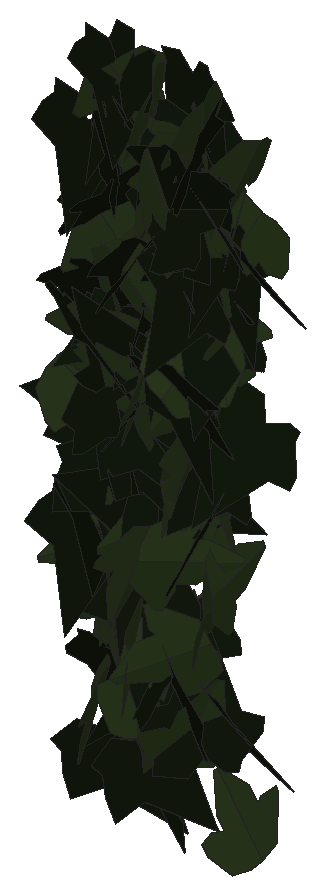
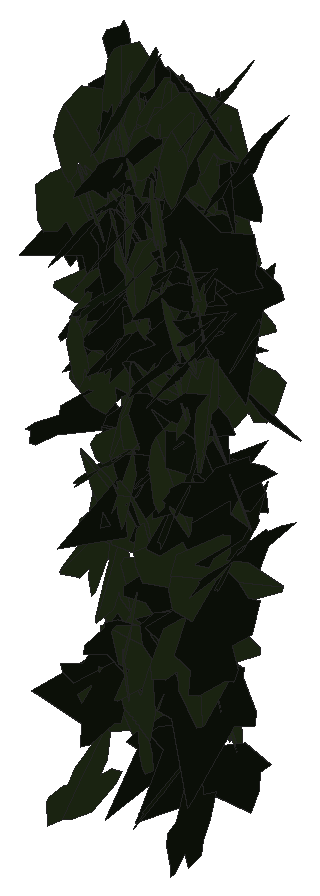
# SketchUp Ruby script. Lengths in inches.
U = 1.inch
M = Sketchup.active_model
def pt(a) = Geom::Point3d.new(a.map { |v| v * U })
def face(e, loops, mat)
  f = e.add_face(loops[0].map { |a| pt(a) })
  loops[1..].each { |l| e.add_face(l.map { |a| pt(a) }).erase! }
  f.material = f.back_material = mat if mat
  f
end
# faces: each face lists its corners as indices into pts; further lists are holes
def faces(e, pts, list, mat = nil) = list.each { |f| face(e, (f[0].is_a?(Array) ? f : [f]).map { |l| l.map { |i| pts[i] } }, mat) }
# xy, xz, yz: faces in a plane at the given z, y or x. An outline is a flat list of corners, or four numbers for a rectangle; further outlines are holes
def ring(l) = l.size == 4 ? [[l[0], l[1]], [l[2], l[1]], [l[2], l[3]], [l[0], l[3]]] : l.each_slice(2).to_a
def flat(e, list, mat, &to3) = list.each { |f| face(e, (f[0].is_a?(Array) ? f : [f]).map { |l| ring(l).map { |u, v| to3.(u, v) } }, mat) }
def xy(e, z, list, mat = nil) = flat(e, list, mat) { |x, y| [x, y, z] }
def xz(e, y, list, mat = nil) = flat(e, list, mat) { |x, z| [x, y, z] }
def yz(e, x, list, mat = nil) = flat(e, list, mat) { |y, z| [x, y, z] }
def lines(e, pts, list) = list.each { |a, b| e.add_line(pt(pts[a]), pt(pts[b])) }
# prism: a flat outline (further loops are holes) pulled along v
def prism(e, loops, v, mat = nil)
  f = face(e, loops, mat); d = Geom::Vector3d.new(v.map { |x| x * U })
  f.pushpull(f.normal.samedirection?(d) ? d.length : -d.length)
end
def box(e, o, s, mat = nil) = prism(e, [[o, [o[0] + s[0], o[1], o[2]], [o[0] + s[0], o[1] + s[1], o[2]], [o[0], o[1] + s[1], o[2]]]], [0, 0, s[2]], mat)
def at(x, y, z, deg = 0) = Geom::Transformation.translation(pt([x, y, z])) * Geom::Transformation.rotation(ORIGIN, Z_AXIS, deg.degrees)
def axes(o, x, y, z) = Geom::Transformation.new([*x, 0, *y, 0, *z, 0, *pt(o).to_a, 1])
def part(name) = M.definitions.add(name)
# library, detail: a bought-in or finely detailed component or shape, given as its bounding box
def library(name, o, s) = part(name).tap { |d| box(d.entities, o, s) }
def detail(e, o, s) = box(e.add_group.entities, o, s)
def put(e, d, t, mat = nil) = e.add_instance(d, t).tap { |i| i.material = mat if mat }
def group(e, t, mat = nil) = e.add_group.tap { |g| g.transformation = t; g.material = mat if mat }.entities
root = M.entities
M.materials.add("efeu1").color = [18, 25, 13]
M.materials.add("efeu2").color = [43, 57, 29]
c1 = part("ivyleaf_10")
p = [[0,0.5,-0.03],[-0.0625,2.02,-0.43],[-0.19,2.01,-0.46],[-0.54,1.05,-0.29],[-0.52,0.625,-0.18],[-0.83,0.76,-0.28],
  [-1.16,0.64,-0.33],[-1.15,0.33,-0.24],[-0.77,-0.39,0.02],[-0.3,-0.51,0.16],[0.04,-0.48,0.23],[-0.02,2.01,-0.4375],
  [-0.06,2.01,-0.43],[0.04,-0.49,0.23],[0.67,-0.49,0.14],[1.38,0.36,-0.2],[1.375,0.51,-0.24],[0.81,0.65,-0.19],
  [0.62,0.59,-0.15],[0.6,1.09,-0.28],[0.5,1.23,-0.31]]
faces(c1.entities,p,[[0,1,2,3,4,5,6,7,8,9,10],[11,12,0,13,14,15,16,17,18,19,20]],"efeu2")
c2 = part("ivyleaf_9")
p = [[1.54,2.16,1.25],[1.36,2.04,1.19],[-0.21,0.99,0.68],[-0.71,1.11,0.82],[-0.85,0.86,0.67],[-0.8,0.17,0.21],
  [-0.9,-0.01,0.1],[-0.67,-0.16,-0.02],[-0.08,-0.08,-0.05],[-0.03,-0.6,-0.4],[0.65,-0.88,-0.66],[0.83,-0.6,-0.49],
  [1.29,-0.42,-0.43],[1.8125,-0.07,-0.26],[1.21,0.44,0.15]]
faces(c2.entities,p,[[0,1,2,3,4,5,6,7,8,9,10,11,12,13,14]],"efeu1")
put(root,c1,axes([25.92,223.86,216.84],[-0.09264,-0.02224,0.49084],[-0.23134,-0.43869,-0.06354],[0.43347,-0.23887,0.07099]))
put(root,c2,axes([25.3,224.02,216.3125],[0.30495,-0.20069,0.34166],[0.2981,-0.16782,-0.36465],[0.26104,0.4261,0.01729]))
put(root,c1,axes([25.88,223.6875,219.36],[-0.37666,0.25048,0.21305],[-0.18134,0.11202,-0.45229],[-0.27431,-0.41799,0.00646]))
put(root,c2,axes([25.625,223.57,217.05],[-0.07559,-0.47947,0.11996],[0.00181,-0.12162,-0.48498],[0.49425,-0.07289,0.02013]))
put(root,c2,axes([25.65,224.01,218.25],[-0.14085,-0.47505,-0.06702],[0.02033,0.06387,-0.49549],[0.47932,-0.1423,0.00132]))
put(root,c2,axes([25.6,223.5,222.08],[0.01946,-0.45872,0.19799],[-0.01144,-0.1985,-0.45877],[0.49949,0.01332,-0.01821]))
put(root,c1,axes([25.62,223.44,217.71],[0.39091,-0.27001,-0.15584],[0.13229,-0.08265,0.47504],[-0.28229,-0.41263,0.00682]))
put(root,c1,axes([25.9,223.83,216.08],[-0.29931,-0.40022,0.01555],[-0.00929,-0.01247,-0.49976],[0.40041,-0.29945,0.00003]))
put(root,c2,axes([25.69,223.82,220.875],[-0.28485,0.05445,0.4073],[0.37648,-0.16405,0.28523],[0.16469,0.46917,0.05246]))
put(root,c2,axes([25.61,223.53,217.14],[0.09476,-0.35196,0.34226],[0.0888,-0.33054,-0.3645],[0.48284,0.12987,-0.00014]))
put(root,c2,axes([25.72,224.27,213.65],[-0.14512,-0.03935,0.47685],[0.10819,-0.4881,-0.00735],[0.46608,0.10104,0.15019]))
put(root,c2,axes([25.9,223.6,215.45],[0.37979,0.21595,-0.24315],[-0.21529,-0.11324,-0.43684],[-0.24374,0.43651,0.00697]))
put(root,c2,axes([26.05,223.25,220.45],[0.16703,0.37187,-0.28951],[-0.19296,-0.22627,-0.40196],[-0.42996,0.24601,0.06793]))
put(root,c1,axes([25.74,223.08,219.14],[0.21945,0.31613,0.31922],[0.11666,0.30299,-0.38025],[-0.43386,0.24137,0.05923]))
put(root,c1,axes([25.95,223.31,215.2],[0.24757,-0.43141,0.05097],[0.02373,-0.04514,-0.49739],[0.43376,0.2487,-0.00187]))
put(root,c2,axes([26.36,223.02,219.06],[-0.32886,0.23102,0.29746],[-0.26211,0.14319,-0.40099],[-0.27046,-0.41967,0.02693]))
put(root,c1,axes([25.99,223.97,222.44],[-0.01091,-0.44648,0.2248],[0.04308,-0.22486,-0.4445],[0.49802,0.00967,0.04338]))
put(root,c2,axes([25.69,223.09,220.02],[0.39503,-0.30608,0.01632],[0.01447,-0.00797,-0.49973],[0.30617,0.39529,0.00256]))
put(root,c2,axes([26.26,223.05,222.3125],[0.07939,0.0261,-0.49297],[-0.49223,0.04213,-0.07704],[0.03752,0.49754,0.03239]))
put(root,c1,axes([25.94,223.7,222.73],[-0.29531,-0.32227,-0.24277],[0.16607,0.1771,-0.4371],[0.36771,-0.3388,0.00244]))
put(root,c1,axes([26.03,223.42,220.59],[-0.25135,0.42248,0.09129],[-0.05371,0.07425,-0.49153],[-0.42888,-0.2569,0.00806]))
put(root,c1,axes([26.05,223.84,220.99],[0.3085,-0.38628,-0.07493],[-0.03814,0.06541,-0.49423],[0.39163,0.31066,0.0109]))
put(root,c2,axes([25.83,224.07,219.8125],[0.07503,-0.48177,0.11074],[0.01907,-0.1091,-0.48758],[0.49397,0.07739,0.002]))
put(root,c2,axes([25.86,223.98,220.7],[0.02957,-0.45823,-0.19786],[0.0326,0.19956,-0.45729],[0.49806,0.01414,0.04168]))
put(root,c1,axes([26.02,224.14,220.49],[0.23063,-0.41696,0.15151],[0.07045,-0.13417,-0.47648],[0.43801,0.24113,-0.00314]))
put(root,c2,axes([26.1,223.83,217.34],[0.37924,-0.03383,0.32409],[-0.32081,0.04835,0.38045],[-0.05708,-0.49651,0.01496]))
put(root,c2,axes([26.09,223.71,222.96],[-0.4266,0.00649,-0.26071],[0.26023,-0.02229,-0.42636],[-0.01716,-0.49946,0.01564]))
put(root,c2,axes([25.86,223.76,222.76],[0.02824,-0.4353,0.24438],[0.07206,-0.23865,-0.43342],[0.49397,0.0597,0.04926]))
put(root,c1,axes([26.2,223.11,219.92],[-0.45447,-0.18164,0.10227],[-0.08785,-0.05557,-0.48908],[0.18904,-0.46251,0.0186]))
put(root,c2,axes([26.26,224.04,219.85],[-0.33124,-0.26273,0.26693],[-0.18906,-0.19032,-0.42194],[0.32332,-0.38046,0.02674]))
put(root,c1,axes([26.15,224.08,218.45],[0.0985,-0.48186,0.09004],[0.01335,-0.08917,-0.4918],[0.49002,0.09929,-0.0047]))
put(root,c2,axes([25.96,224.16,217.85],[0.02168,-0.23686,0.4398],[0.05246,-0.4367,-0.23778],[0.49677,0.05645,0.00592]))
put(root,c1,axes([26.07,223.32,221.05],[-0.23934,-0.38368,-0.21332],[0.20248,0.11909,-0.44138],[0.38951,-0.29766,0.09837]))
put(root,c2,axes([25.93,223.46,214.49],[-0.09453,-0.15668,-0.46531],[0.22631,0.40661,-0.1829],[0.43572,-0.24518,-0.00596]))
put(root,c1,axes([25.88,223.52,216.28],[0.1338,-0.13367,0.46285],[0.40176,-0.23413,-0.18376],[0.26586,0.42109,0.04475]))
put(root,c2,axes([26.1,224.24,219.74],[-0.12442,-0.41104,0.25605],[-0.01447,-0.2611,-0.42617],[0.48405,-0.11346,0.05308]))
put(root,c2,axes([26.33,223.99,220.51],[-0.38732,-0.29247,0.12021],[-0.08899,-0.08158,-0.48521],[0.30343,-0.39725,0.01114]))
put(root,c2,axes([26.28,222.98,221.65],[0.11209,0.48323,0.06269],[0.01307,0.06132,-0.49605],[-0.4871,0.11284,0.00112]))
put(root,c2,axes([26.04,223.44,218.04],[-0.17073,-0.30697,-0.35584],[0.1756,0.3095,-0.35125],[0.43591,-0.24491,0.00213]))
put(root,c2,axes([25.92,223.86,222.29],[0.36282,-0.33171,0.09129],[0.06779,-0.06114,-0.4916],[0.3373,0.36909,0.00061]))
put(root,c1,axes([26.4,223.13,219.41],[-0.46056,-0.14243,0.13267],[-0.12576,-0.04237,-0.48207],[0.14857,-0.47741,0.0032]))
put(root,c2,axes([26.43,223.75,217.41],[-0.01959,-0.017,0.49933],[-0.41095,-0.28365,-0.02578],[0.28415,-0.4114,-0.00286]))
put(root,c1,axes([26.46,223.62,222.21],[-0.44911,-0.17426,0.13391],[-0.1138,-0.07624,-0.48087],[0.18801,-0.46241,0.02882]))
put(root,c2,axes([26.07,224,214.35],[0.21511,-0.45076,0.02334],[0.01062,-0.0208,-0.49945],[0.45124,0.21537,0.00062]))
put(root,c1,axes([26.39,223.86,220.82],[-0.07417,-0.47008,0.15338],[0.01785,-0.15754,-0.4742],[0.49415,-0.06487,0.04015]))
put(root,c1,axes([26.05,223.64,214.33],[-0.18337,0.00872,0.46508],[0.43547,-0.17253,0.17493],[0.16353,0.46921,0.05568]))
put(root,c2,axes([26.23,223.35,218.46],[-0.04078,0.49826,0.00887],[-0.00261,-0.00912,0.49991],[0.49833,0.04072,0.00335]))
put(root,c1,axes([26.41,223.96,217.15],[-0.02506,0.01961,0.49899],[0.01468,-0.49937,0.02036],[0.49916,0.01567,0.02446]))
put(root,c1,axes([26.46,223.56,222.65],[0.09237,-0.40977,-0.27122],[-0.02638,0.27144,-0.41908],[0.49068,0.09173,0.02852]))
put(root,c2,axes([26.28,223.91,218.97],[-0.19526,-0.37314,-0.26952],[0.11483,0.24402,-0.42103],[0.44574,-0.22632,-0.0096]))
put(root,c1,axes([26.46,223.52,218.66],[-0.33117,0.37288,0.03585],[0.02405,-0.02659,0.49871],[0.37383,0.33204,-0.00032]))
put(root,c2,axes([26.57,223.3,219.23],[0.25555,0.00267,0.42975],[-0.42824,0.04361,0.25438],[-0.03612,-0.49809,0.02457]))
put(root,c2,axes([26.34,223.63,216.52],[-0.32198,-0.29113,-0.24814],[0.17468,0.17665,-0.43391],[0.34032,-0.36611,-0.01205]))
put(root,c1,axes([26.47,223.8,221.51],[0.16813,-0.45372,-0.12599],[-0.04098,0.11917,-0.48386],[0.4691,0.17303,0.00289]))
put(root,c2,axes([26.68,223.45,215.59],[-0.43694,0.2318,-0.07316],[0.06226,-0.03874,-0.49459],[-0.23496,-0.44132,0.00498]))
put(root,c1,axes([26.31,223.52,215.95],[0.23028,-0.31621,0.31142],[0.21559,-0.22696,-0.38988],[0.38793,0.31385,0.03181]))
put(root,c1,axes([26.47,223.41,219.17],[0.23988,-0.43815,0.02189],[0.00612,-0.0216,-0.4995],[0.43866,0.2399,-0.005]))
put(root,c2,axes([26.625,223.01,220.82],[-0.0202,0.45126,0.21438],[0.00085,0.21459,-0.45161],[-0.49959,-0.01788,-0.00944]))
put(root,c1,axes([26.53,223.33,217.15],[0.01692,-0.46884,0.17292],[0.01414,-0.1725,-0.46909],[0.49951,0.02076,0.00743]))
put(root,c1,axes([26.55,223.16,215.08],[-0.01082,0.46922,-0.17239],[-0.00378,0.17235,0.46934],[0.49987,0.01146,-0.00019]))
put(root,c2,axes([26.29,223.58,218.33],[0.2317,-0.39063,-0.20909],[-0.0385,0.21731,-0.44866],[0.4414,0.22401,0.07062]))
put(root,c1,axes([26.54,224.07,220.61],[0.15258,-0.38364,0.28203],[0.10313,-0.2625,-0.41287],[0.46485,0.18416,-0.00098]))
put(root,c1,axes([26.625,223.44,221.58],[-0.47344,0.15701,-0.03462],[0.03459,-0.00567,-0.49877],[-0.15702,-0.47467,-0.00549]))
put(root,c2,axes([26.47,223.36,214.57],[0.12144,-0.26162,-0.40842],[-0.07568,0.40565,-0.28235],[0.47909,0.13039,0.05893]))
put(root,c2,axes([26.79,223.17,221.09],[0.04507,0.44037,-0.23248],[-0.03539,-0.23001,-0.44254],[-0.49671,0.05635,0.01043]))
put(root,c2,axes([26.36,224.09,220.58],[0.10427,-0.31253,0.3761],[0.16457,-0.3397,-0.3279],[0.46049,0.19217,0.03202]))
put(root,c1,axes([26.48,223.04,220.85],[-0.40393,0.0784,-0.28407],[0.27901,-0.0534,-0.41147],[-0.09486,-0.49092,-0.00061]))
put(root,c2,axes([26.5,223.45,218.78],[0.00831,-0.34951,-0.35746],[0.05502,0.35597,-0.34678],[0.49689,-0.03357,0.04437]))
put(root,c2,axes([26.51,223.9,219.87],[0.13072,-0.44339,-0.19057],[-0.02937,0.18976,-0.46166],[0.48172,0.13189,0.02357]))
put(root,c2,axes([26.46,223.61,217.76],[0.04818,-0.01555,-0.49743],[0.1009,0.48968,-0.00554],[0.48734,-0.09985,0.05032]))
put(root,c1,axes([26.37,224.14,214.84],[0.01469,-0.07094,0.49472],[0.46274,-0.18507,-0.04027],[0.18883,0.45904,0.06022]))
put(root,c2,axes([26.625,223.94,216.01],[-0.21428,-0.41987,-0.16672],[0.0709,0.15098,-0.47136],[0.44616,-0.22564,-0.00517]))
put(root,c1,axes([26.67,223.54,215.5],[0.14754,0.28275,-0.38508],[0.12259,0.36712,0.31653],[0.46174,-0.18781,0.039]))
put(root,c1,axes([26.62,224.05,218.85],[-0.10077,-0.03125,0.48874],[0.2207,-0.44834,0.01684],[0.43719,0.21913,0.10415]))
put(root,c1,axes([27.11,224.12,219.45],[-0.13771,-0.10106,0.46992],[-0.37913,-0.27764,-0.17081],[0.29546,-0.40337,-0.00016]))
put(root,c2,axes([26.6,223.5,220.09],[-0.01149,-0.04789,-0.49757],[0.1108,0.48508,-0.04924],[0.48743,-0.11139,-0.00054]))
put(root,c1,axes([26.87,223.49,221.99],[0.03217,-0.44888,0.21788],[-0.00197,-0.21844,-0.44975],[0.49896,0.02808,-0.01582]))
put(root,c2,axes([26.64,223.91,219.78],[0.05427,-0.47739,-0.13839],[0.00108,0.13932,-0.4802],[0.49705,0.05182,0.01615]))
put(root,c1,axes([26.72,224.07,219.0625],[-0.125,0.33887,-0.34574],[0.07489,-0.33925,-0.35958],[-0.4783,-0.14168,0.03406]))
put(root,c2,axes([26.79,224.35,220.42],[-0.21873,-0.28318,0.34923],[0.02701,-0.39594,-0.30414],[0.44881,-0.11419,0.1885]))
put(root,c2,axes([26.7,224.11,222.15],[-0.02224,-0.49506,-0.06647],[0.01144,0.06602,-0.49549],[0.49937,-0.02356,0.00839]))
put(root,c2,axes([26.7,223.93,220.4],[0.1171,-0.4854,-0.02586],[-0.00057,0.02647,-0.4993],[0.48609,0.11697,0.00565]))
put(root,c1,axes([26.63,224.18,215.75],[0.02832,-0.10785,0.48741],[0.39932,-0.28807,-0.08694],[0.29957,0.39419,0.06982]))
put(root,c1,axes([27.21,223.375,216.03],[-0.1742,-0.13423,0.44904],[-0.3376,-0.29636,-0.21955],[0.32509,-0.37968,0.01262]))
put(root,c2,axes([27.03,223.6,220.99],[-0.14488,0.33229,-0.34438],[0.13202,-0.3181,-0.36247],[-0.45998,-0.19596,0.00443]))
put(root,c1,axes([27.04,222.9,222.27],[-0.11141,0.44621,0.19617],[-0.12853,0.16721,-0.45334],[-0.47018,-0.15144,0.07745]))
put(root,c2,axes([26.73,224.02,222.83],[0.22354,-0.43653,0.09733],[0.03063,-0.09361,-0.4902],[0.4462,0.22512,-0.01511]))
put(root,c1,axes([26.67,224.05,217.39],[0.25981,-0.13375,-0.40572],[0.37364,-0.15906,0.2917],[-0.2071,-0.45477,0.0173]))
put(root,c2,axes([26.79,223.85,221.19],[0.27173,-0.39147,-0.15138],[-0.04405,0.15274,-0.47406],[0.4174,0.27097,0.04852]))
put(root,c1,axes([27,223.7,222.23],[0.23688,-0.42763,0.10497],[0.05135,-0.09155,-0.48886],[0.43732,0.24238,0.00055]))
put(root,c1,axes([26.91,223.96,218.03],[-0.36664,0.27092,-0.20537],[0.16535,-0.12181,-0.45588],[-0.29705,-0.4022,-0.00027]))
put(root,c1,axes([27.19,223.08,218.3],[-0.07843,0.1704,0.46348],[-0.24243,0.39556,-0.18645],[-0.43021,-0.25396,0.02058]))
put(root,c2,axes([27.51,223.08,221.58],[-0.2086,0.23029,0.39173],[-0.32546,0.22509,-0.30564],[-0.31712,-0.38249,0.05599]))
put(root,c1,axes([27.45,223.69,221.12],[-0.14269,0.09933,0.4688],[-0.44746,0.14745,-0.16744],[-0.17151,-0.46732,0.04681]))
put(root,c2,axes([27.04,224.03,218.04],[-0.18763,-0.36123,0.29036],[0.05837,-0.32917,-0.3718],[0.45977,-0.10562,0.16569]))
put(root,c2,axes([27.41,223.01,222.31],[0.14569,0.22809,-0.42042],[-0.35729,-0.24029,-0.25418],[-0.318,0.37448,0.09297]))
put(root,c1,axes([27.08,223.45,214.67],[-0.23879,-0.42136,0.12424],[0.06966,0.1033,0.48423],[-0.43374,0.24857,0.00937]))
put(root,c2,axes([26.8,224.1,220.2],[0.34827,-0.05313,-0.3548],[0.35697,0.00194,0.3501],[-0.03582,-0.49717,0.03928]))
put(root,c1,axes([27.28,223.68,221.84],[-0.31596,0.38633,-0.03037],[-0.02346,0.02005,0.49905],[0.38681,0.31678,0.00546]))
put(root,c1,axes([27.01,223.03,217.27],[-0.09955,-0.09895,-0.47989],[0.33561,0.34302,-0.14035],[0.35701,-0.35006,-0.00188]))
put(root,c2,axes([27.05,222.99,219.64],[0.49215,0.03911,-0.07912],[-0.07866,-0.00893,-0.49369],[-0.04003,0.49839,-0.00264]))
put(root,c2,axes([27.32,223.45,214.75],[-0.44958,-0.08826,0.20022],[0.20247,0.00567,0.45714],[-0.08297,0.49212,0.03064]))
put(root,c1,axes([27.33,223.45,216.53],[0.03554,-0.1944,-0.45929],[-0.07934,0.45239,-0.19761],[0.49238,0.08692,0.00131]))
put(root,c1,axes([27.16,223.39,218.57],[0.14426,-0.39282,0.27365],[0.13311,-0.24163,-0.41701],[0.45986,0.19316,0.03486]))
put(root,c1,axes([27.27,223.44,222.79],[0.04447,-0.483,-0.12139],[0.02082,0.12357,-0.48404],[0.49758,0.038,0.03111]))
put(root,c2,axes([27.22,223.51,220.6875],[-0.11867,-0.42543,0.23436],[-0.0748,-0.22237,-0.44154],[0.47992,-0.13986,-0.01087]))
put(root,c1,axes([27.1875,223.05,219.57],[0.20951,0.18799,-0.41324],[0.12637,0.41298,0.25194],[0.43605,-0.21001,0.12553]))
put(root,c2,axes([27.01,223.4375,215.25],[0.02413,-0.1325,0.48152],[0.19591,-0.44093,-0.13115],[0.45939,0.195,0.03063]))
put(root,c2,axes([27.03,223.34,219.34],[0.20332,-0.44617,0.09792],[0.05276,-0.08353,-0.49014],[0.45374,0.20964,0.01311]))
put(root,c1,axes([27.28,224.16,219.75],[0.10387,-0.45555,0.17799],[0.07236,-0.16564,-0.46618],[0.48371,0.12261,0.03152]))
put(root,c2,axes([27.21,223.89,220.01],[-0.1058,-0.48316,0.07326],[-0.00188,-0.07456,-0.49441],[0.48868,-0.10489,0.01396]))
put(root,c2,axes([27.42,222.97,217.36],[0.03382,0.28484,0.40954],[0.01927,0.40943,-0.28635],[-0.49848,0.03515,0.01672]))
put(root,c1,axes([27.19,223.7,220.06],[0.43332,0.21415,0.12795],[0.09367,0.098,-0.48127],[-0.23121,0.44106,0.04481]))
put(root,c1,axes([27.18,223.63,221.24],[-0.32466,0.19903,-0.32401],[0.22458,-0.24344,-0.37457],[-0.30686,-0.38875,0.06867]))
put(root,c2,axes([27.59,222.92,222.58],[-0.13876,0.1211,-0.46484],[-0.3592,0.29509,0.18411],[0.31893,0.38504,0.00511]))
put(root,c1,axes([27.43,223.59,216.82],[0.06221,-0.00606,-0.49608],[0.02192,0.49951,-0.00335],[0.49563,-0.02133,0.06241]))
put(root,c2,axes([27.07,223.69,221.64],[0.18132,-0.32196,0.33684],[0.19603,-0.2752,-0.36856],[0.42273,0.26571,0.02643]))
put(root,c1,axes([27.65,223.93,221.31],[-0.42703,-0.04645,0.25591],[-0.22722,-0.17277,-0.41051],[0.12656,-0.4669,0.12645]))
put(root,c2,axes([27.05,223.88,215.06],[0.35836,-0.25137,0.24164],[0.19908,-0.13697,-0.43773],[0.28626,0.40994,0.00191]))
put(root,c1,axes([27.4,223.92,221.42],[0.32034,-0.37726,0.0711],[0.04911,-0.05157,-0.4949],[0.38075,0.32406,0.00402]))
put(root,c2,axes([27.49,223.57,221.28],[-0.4262,0.03758,-0.25873],[0.25648,-0.03587,-0.4277],[-0.05071,-0.49729,0.0113]))
put(root,c1,axes([27.56,223.97,213.45],[-0.00237,0.48787,0.10945],[-0.02126,-0.10946,0.48741],[0.49954,-0.00235,0.02126]))
put(root,c2,axes([27.51,224.23,218.59],[-0.25849,-0.39844,0.1563],[-0.04812,-0.15438,-0.47313],[0.42529,-0.25964,0.04147]))
put(root,c2,axes([27.32,223.87,221.05],[0.12696,-0.4824,-0.03428],[-0.00753,0.03346,-0.49882],[0.48355,0.12718,0.00123]))
put(root,c2,axes([27.22,223.78,221.16],[0.45152,-0.19134,0.09754],[0.08693,-0.04483,-0.49034],[0.19639,0.45976,-0.00722]))
put(root,c1,axes([27.6,223.88,222.18],[0.03881,-0.45934,0.19364],[0.00024,-0.19421,-0.46074],[0.49849,0.03585,-0.01485]))
